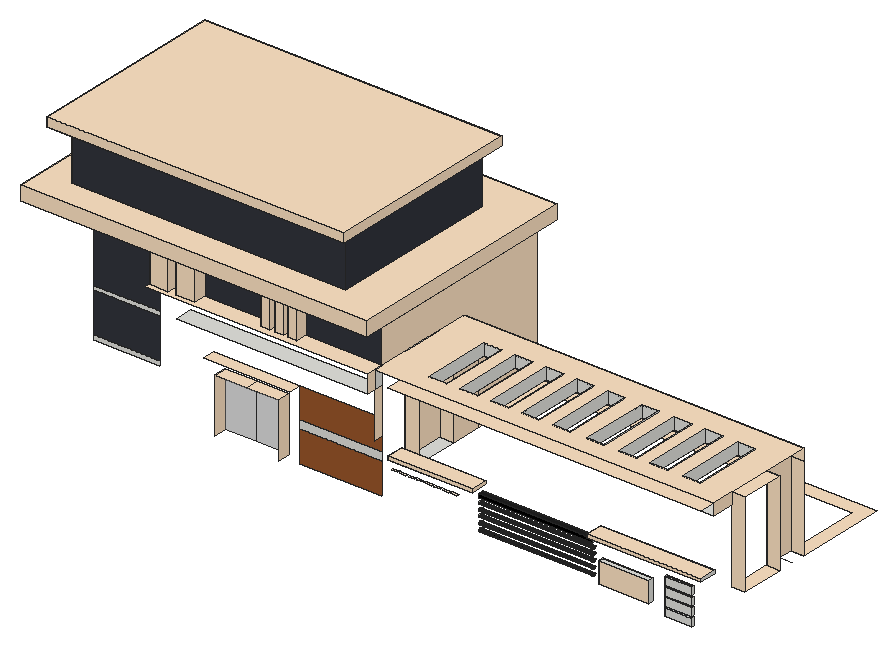
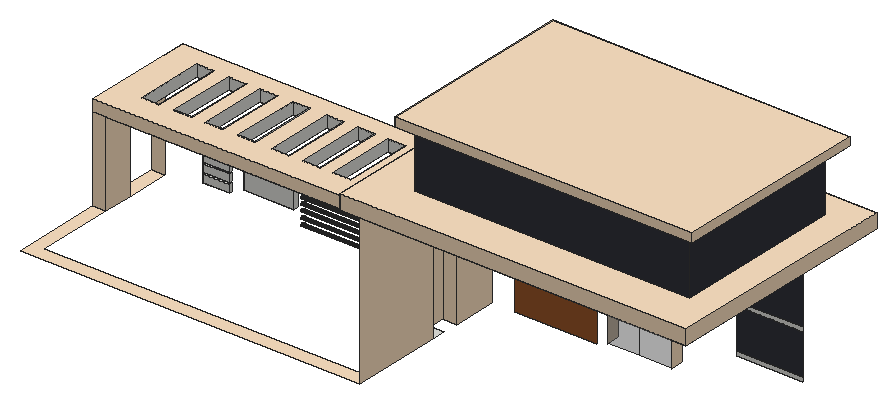
# SketchUp Ruby script. Lengths in inches.
U = 1.inch
M = Sketchup.active_model
def pt(a) = Geom::Point3d.new(a.map { |v| v * U })
def face(e, loops, mat)
  f = e.add_face(loops[0].map { |a| pt(a) })
  loops[1..].each { |l| e.add_face(l.map { |a| pt(a) }).erase! }
  f.material = f.back_material = mat if mat
  f
end
# faces: each face lists its corners as indices into pts; further lists are holes
def faces(e, pts, list, mat = nil) = list.each { |f| face(e, (f[0].is_a?(Array) ? f : [f]).map { |l| l.map { |i| pts[i] } }, mat) }
# xy, xz, yz: faces in a plane at the given z, y or x. An outline is a flat list of corners, or four numbers for a rectangle; further outlines are holes
def ring(l) = l.size == 4 ? [[l[0], l[1]], [l[2], l[1]], [l[2], l[3]], [l[0], l[3]]] : l.each_slice(2).to_a
def flat(e, list, mat, &to3) = list.each { |f| face(e, (f[0].is_a?(Array) ? f : [f]).map { |l| ring(l).map { |u, v| to3.(u, v) } }, mat) }
def xy(e, z, list, mat = nil) = flat(e, list, mat) { |x, y| [x, y, z] }
def xz(e, y, list, mat = nil) = flat(e, list, mat) { |x, z| [x, y, z] }
def yz(e, x, list, mat = nil) = flat(e, list, mat) { |y, z| [x, y, z] }
def lines(e, pts, list) = list.each { |a, b| e.add_line(pt(pts[a]), pt(pts[b])) }
# prism: a flat outline (further loops are holes) pulled along v
def prism(e, loops, v, mat = nil)
  f = face(e, loops, mat); d = Geom::Vector3d.new(v.map { |x| x * U })
  f.pushpull(f.normal.samedirection?(d) ? d.length : -d.length)
end
def box(e, o, s, mat = nil) = prism(e, [[o, [o[0] + s[0], o[1], o[2]], [o[0] + s[0], o[1] + s[1], o[2]], [o[0], o[1] + s[1], o[2]]]], [0, 0, s[2]], mat)
def at(x, y, z, deg = 0) = Geom::Transformation.translation(pt([x, y, z])) * Geom::Transformation.rotation(ORIGIN, Z_AXIS, deg.degrees)
def axes(o, x, y, z) = Geom::Transformation.new([*x, 0, *y, 0, *z, 0, *pt(o).to_a, 1])
def part(name) = M.definitions.add(name)
# library, detail: a bought-in or finely detailed component or shape, given as its bounding box
def library(name, o, s) = part(name).tap { |d| box(d.entities, o, s) }
def detail(e, o, s) = box(e.add_group.entities, o, s)
def put(e, d, t, mat = nil) = e.add_instance(d, t).tap { |i| i.material = mat if mat }
def group(e, t, mat = nil) = e.add_group.tap { |g| g.transformation = t; g.material = mat if mat }.entities
root = M.entities
M.materials.add("[0012_Bisque]").color = [255, 228, 196]
M.materials.add("[0028_AntiqueWhite]").color = [250, 235, 215]
M.materials.add("[Color M08]").color = [30, 30, 30]
M.materials.add("[Color M09]").color = [0, 0, 0]
M.materials.add("[Formica Laminate Dark]").color = [50, 53, 60]
M.materials.add("[Translucent Glass Gray]").color = [128, 128, 128]
M.materials["[Translucent Glass Gray]"].alpha = 0.5
M.materials.add("[Wood Cherry Original]").color = [152, 86, 42]
box(root,[407.7,39.05,294.93],[17.88,1.62,5])
box(root,[407.7,39.05,301.12],[17.88,1.62,5])
box(root,[407.7,39.05,307.12],[17.88,1.62,5])
box(root,[407.7,39.05,313.43],[17.88,1.62,5])
xy(root,300,[[365.58,37.23,398.96,40.67]])
xy(root,308.625,[[215,65.9,223.75,94.79],[215,105.21,223.75,114.71]])
xy(root,308.625,[[430.46,65.9,439.21,94.79],[215,114.71,223.75,114.71,223.75,165.7,430.46,165.7,430.46,114.71,439.21,114.71,439.21,174.44,215,174.44]],"[0012_Bisque]")
xy(root,313.68,[[365.58,37.23,398.96,40.67]])
xy(root,317.125,[[[279.65,45.65,355.06,49.39],[330.07,45.65,330.29,45.68,330.5,45.77,330.68,45.91,330.82,46.09,330.91,46.3,330.94,46.53,330.91,46.75,330.82,46.96,330.68,47.15,330.5,47.29,330.29,47.37,330.07,47.4,329.84,47.37,329.63,47.29,329.45,47.15,329.31,46.96,329.22,46.75,329.19,46.53,329.22,46.3,329.31,46.09,329.45,45.91,329.63,45.77,329.84,45.68],[305.63,45.65,305.85,45.68,306.07,45.77,306.25,45.91,306.39,46.09,306.47,46.3,306.5,46.53,306.47,46.75,306.39,46.96,306.25,47.15,306.07,47.29,305.85,47.37,305.63,47.4,305.4,47.37,305.19,47.29,305.01,47.15,304.87,46.96,304.78,46.75,304.75,46.53,304.78,46.3,304.87,46.09,305.01,45.91,305.19,45.77,305.4,45.68]]],"[Color M08]")
xy(root,317.98,[[227.14,39.36,231.39,40.67],[232.64,39.36,236.89,40.67],[238.51,39.36,242.76,40.67],[244.08,39.36,248.33,40.67],[249.76,39.36,254.01,40.67],
  [255.33,39.36,259.58,40.67],[260.95,39.36,265.2,40.67],[266.39,39.36,270.64,40.67]],"[0028_AntiqueWhite]")
xy(root,319.4375,[[279.65,45.65,355.06,49.39]],"[Color M08]")
xy(root,322.3125,[[223.75,40.67,279.65,51.97],[355.06,40.67,430.46,51.97]])
xy(root,324.5,[[223.75,40.67,279.65,51.97],[355.06,40.67,430.46,51.97]],"[0012_Bisque]")
xy(root,333.89,[[111.55,38.36,132.61,46.73],[132.61,38.36,153.67,46.73]],"[0012_Bisque]")
xy(root,341.36,[[104.08,38.36,161.14,46.73]],"[0012_Bisque]")
xy(root,360.6,[[89.06,35.36,215,46.73]])
xy(root,364.53,[[430.46,40.67,439.21,55.48]])
xy(root,364.53,[[[223.75,40.67,223.75,65.9,215,65.9,215,94.79,223.75,94.79,223.75,114.71,430.46,114.71,430.46,94.79,439.21,94.79,439.21,65.9,430.46,65.9,430.46,40.67],[241.35,52.73,252.92,98.23],[408.67,52.73,420.23,98.23],[261.85,52.73,273.42,98.23],[387.17,52.73,398.73,98.23],[282.29,52.73,293.85,98.23],[366.79,52.73,378.35,98.23],[302.29,52.73,313.85,98.23],[345.29,52.73,356.85,98.23],[322.73,52.73,334.29,98.23]]],"[0012_Bisque]")
xy(root,372.25,[[68.38,38.48,80.44,46.73],[85.88,38.48,97.94,46.73],[140.45,39.92,146.58,46.73],[149.51,39.92,155.64,46.73],[158.39,39.92,164.51,46.73]])
xy(root,372.25,[[68.38,35.36,215,35.36,215,46.73,164.51,46.73,164.51,39.92,158.39,39.92,158.39,46.73,155.64,46.73,155.64,39.92,149.51,39.92,149.51,46.73,146.58,46.73,146.58,39.92,140.45,39.92,140.45,46.73,97.94,46.73,97.94,38.48,85.88,38.48,85.88,46.73,80.44,46.73,80.44,38.48,68.38,38.48],[[215,40.67,439.21,114.71],[241.35,52.73,252.92,98.23],[261.85,52.73,273.42,98.23],[282.29,52.73,293.85,98.23],[302.29,52.73,313.85,98.23],[322.73,52.73,334.29,98.23],[345.29,52.73,356.85,98.23],[366.79,52.73,378.35,98.23],[387.17,52.73,398.73,98.23],[408.67,52.73,420.23,98.23]]],"[0012_Bisque]")
xy(root,397.4375,[[68.38,38.48,80.44,46.73],[85.88,38.48,97.94,46.73]],"[0012_Bisque]")
xy(root,398.3125,[[140.45,39.92,146.58,46.73],[149.51,39.92,155.64,46.73],[158.39,39.92,164.51,46.73]],"[0012_Bisque]")
xy(root,406.75,[[24.6875,46.73,215,174.44]])
xy(root,406.75,[[0,17.17,228.57,46.73],[0,46.73,24.6875,174.44],[215,46.73,228.57,174.44]],"[0012_Bisque]")
xy(root,416.3125,[[18.79,35.8,200.11,147.86]])
xy(root,416.3125,[[[0,17.17,228.57,174.44],[18.79,35.8,200.11,147.86]]],"[0012_Bisque]")
xy(root,453.1875,[[13.16,22.61,209.05,35.8],[13.16,35.8,18.79,147.86],[18.79,35.8,200.11,147.86],[200.11,35.8,209.05,152.92],[13.16,147.86,200.11,152.92]])
xy(root,459,[[13.16,22.61,209.05,152.92]],"[0012_Bisque]")
xz(root,17.17,[[0,406.75,228.57,416.3125]],"[0012_Bisque]")
xz(root,22.61,[[13.16,453.1875,209.05,459]],"[0012_Bisque]")
xz(root,35.8,[[18.79,416.3125,200.11,453.1875]],"[Formica Laminate Dark]")
xz(root,37.23,[[365.58,300,398.96,313.68]],"[0012_Bisque]")
xz(root,38.48,[[68.38,372.25,80.44,397.4375],[85.88,372.25,97.94,397.4375]],"[0012_Bisque]")
xz(root,39.92,[[140.45,372.25,146.58,398.3125],[149.51,372.25,155.64,398.3125],[158.39,372.25,164.51,398.3125]],"[0012_Bisque]")
xz(root,40.67,[[365.58,300,398.96,313.68]])
xz(root,40.67,[[223.75,322.3125,279.65,324.5],[355.06,322.3125,430.46,324.5]],"[0012_Bisque]")
xz(root,45.65,[[279.65,317.125,355.06,319.4375]],"[Color M09]")
xz(root,46.73,[[161.14,315.73,215,320.89],[24.6875,320.49,68.38,323.52],[24.6875,349.9375,68.38,352.67],[68.38,372.25,80.44,397.4375],[85.88,372.25,97.94,397.4375],
  [140.45,372.25,146.58,398.3125],[149.51,372.25,155.64,398.3125],[158.39,372.25,164.51,398.3125]])
xz(root,46.73,[[24.6875,323.52,68.38,349.9375],[24.6875,352.67,68.38,352.67,68.38,397.4375,80.44,397.4375,80.44,372.25,85.88,372.25,85.88,397.4375,97.94,397.4375,97.94,372.25,140.45,372.25,140.45,398.3125,146.58,398.3125,146.58,372.25,149.51,372.25,149.51,398.3125,155.64,398.3125,155.64,372.25,158.39,372.25,158.39,398.3125,164.51,398.3125,164.51,372.25,215,372.25,215,406.75,24.6875,406.75]],"[Formica Laminate Dark]")
xz(root,46.73,[[111.55,297.86,132.61,333.89],[132.61,297.86,153.67,333.89]],"[Translucent Glass Gray]")
xz(root,46.73,[[161.14,295.26,215,315.73],[161.14,320.89,215,341.36]],"[Wood Cherry Original]")
xz(root,49.39,[[279.65,317.125,355.06,319.4375]],"[Formica Laminate Dark]")
xz(root,51.97,[[223.75,322.3125,279.65,324.5],[355.06,322.3125,430.46,324.5]],"[0012_Bisque]")
xz(root,52.73,[[241.35,364.53,252.92,372.25],[261.85,364.53,273.42,372.25],[282.29,364.53,293.85,372.25],[302.29,364.53,313.85,372.25],[322.73,364.53,334.29,372.25],
  [345.29,364.53,356.85,372.25],[366.79,364.53,378.35,372.25],[387.17,364.53,398.73,372.25],[408.67,364.53,420.23,372.25]])
xz(root,65.9,[[215,308.625,223.75,364.53],[430.46,308.625,439.21,364.53]],"[0012_Bisque]")
xz(root,94.79,[[215,308.625,223.75,364.53],[430.46,308.625,439.21,364.53]],"[0012_Bisque]")
xz(root,98.23,[[241.35,364.53,252.92,372.25],[261.85,364.53,273.42,372.25],[282.29,364.53,293.85,372.25],[302.29,364.53,313.85,372.25],[322.73,364.53,334.29,372.25],
  [345.29,364.53,356.85,372.25],[366.79,364.53,378.35,372.25],[387.17,364.53,398.73,372.25],[408.67,364.53,420.23,372.25]])
xz(root,114.71,[[215,308.625,215,372.25,439.21,372.25,439.21,364.53,223.75,364.53,223.75,308.625],[430.46,308.625,439.21,364.53]],"[0012_Bisque]")
xz(root,147.86,[[18.79,416.3125,200.11,453.1875]],"[Formica Laminate Dark]")
xz(root,152.92,[[13.16,453.1875,209.05,459]],"[0012_Bisque]")
xz(root,174.44,[[0,406.75,228.57,416.3125]],"[0012_Bisque]")
yz(root,0,[[17.17,406.75,174.44,416.3125]],"[0012_Bisque]")
yz(root,13.16,[[22.61,453.1875,152.92,459]],"[0012_Bisque]")
yz(root,18.79,[[35.8,416.3125,147.86,453.1875]],"[Formica Laminate Dark]")
yz(root,68.38,[[38.48,372.25,46.73,397.4375]],"[0012_Bisque]")
yz(root,80.44,[[38.48,372.25,46.73,397.4375]],"[0012_Bisque]")
yz(root,85.88,[[38.48,372.25,46.73,397.4375]],"[0012_Bisque]")
yz(root,97.94,[[38.48,372.25,46.73,397.4375]],"[0012_Bisque]")
yz(root,111.55,[[38.36,297.86,46.73,333.89]],"[0012_Bisque]")
yz(root,140.45,[[39.92,372.25,46.73,398.3125]],"[0012_Bisque]")
yz(root,146.58,[[39.92,372.25,46.73,398.3125]],"[0012_Bisque]")
yz(root,149.51,[[39.92,372.25,46.73,398.3125]],"[0012_Bisque]")
yz(root,153.67,[[38.36,297.86,46.73,333.89]],"[0012_Bisque]")
yz(root,155.64,[[39.92,372.25,46.73,398.3125]],"[0012_Bisque]")
yz(root,158.39,[[39.92,372.25,46.73,398.3125]],"[0012_Bisque]")
yz(root,164.51,[[39.92,372.25,46.73,398.3125]],"[0012_Bisque]")
yz(root,200.11,[[35.8,416.3125,147.86,453.1875]],"[Formica Laminate Dark]")
yz(root,209.05,[[22.61,453.1875,152.92,459]],"[0012_Bisque]")
yz(root,215,[[40.67,360.6,46.73,372.25],[65.9,364.53,94.79,372.25]])
yz(root,215,[[114.71,308.625,174.44,308.625,174.44,406.75,46.73,406.75,46.73,372.25,114.71,372.25],[65.9,308.625,94.79,364.53],[40.67,330.3125,46.73,360.6],[35.36,360.6,40.67,372.25]],"[0012_Bisque]")
yz(root,223.75,[[40.67,322.3125,51.97,324.5]])
yz(root,223.75,[[94.79,308.625,114.71,364.53]],"[0012_Bisque]")
yz(root,228.57,[[17.17,406.75,174.44,416.3125]],"[0012_Bisque]")
yz(root,241.35,[[52.73,364.53,98.23,372.25]])
yz(root,252.92,[[52.73,364.53,98.23,372.25]])
yz(root,261.85,[[52.73,364.53,98.23,372.25]])
yz(root,273.42,[[52.73,364.53,98.23,372.25]])
yz(root,279.65,[[46.99,296.71,46.77,296.74,46.55,296.83,46.375,296.97,46.23,297.15,46.15,297.36,46.12,297.59,46.15,297.8125,46.23,298.02,46.375,298.2,46.55,298.34,46.77,298.43,46.99,298.46,47.22,298.43,47.43,298.34,47.61,298.2,47.75,298.02,47.84,297.8125,47.87,297.59,47.84,297.36,47.75,297.15,47.61,296.97,47.43,296.83,47.22,296.74],[46.99,300.84,46.77,300.87,46.55,300.95,46.375,301.09,46.23,301.27,46.15,301.48,46.12,301.71,46.15,301.9375,46.23,302.15,46.375,302.33,46.55,302.47,46.77,302.56,46.99,302.59,47.22,302.56,47.43,302.47,47.61,302.33,47.75,302.15,47.84,301.9375,47.87,301.71,47.84,301.48,47.75,301.27,47.61,301.09,47.43,300.95,47.22,300.87],[46.99,305.27,46.77,305.3,46.55,305.39,46.375,305.53,46.23,305.71,46.15,305.92,46.12,306.15,46.15,306.375,46.23,306.59,46.375,306.77,46.55,306.91,46.77,306.99,46.99,307.02,47.22,306.99,47.43,306.91,47.61,306.77,47.75,306.59,47.84,306.375,47.87,306.15,47.84,305.92,47.75,305.71,47.61,305.53,47.43,305.39,47.22,305.3],[46.99,308.96,46.77,308.99,46.55,309.08,46.375,309.22,46.23,309.4,46.15,309.61,46.12,309.84,46.15,310.0625,46.23,310.27,46.375,310.45,46.55,310.59,46.77,310.68,46.99,310.71,47.22,310.68,47.43,310.59,47.61,310.45,47.75,310.27,47.84,310.0625,47.87,309.84,47.84,309.61,47.75,309.4,47.61,309.22,47.43,309.08,47.22,308.99],[46.99,313.02,46.77,313.05,46.55,313.14,46.375,313.28,46.23,313.46,46.15,313.67,46.12,313.9,46.15,314.125,46.23,314.34,46.375,314.52,46.55,314.66,46.77,314.74,46.99,314.77,47.22,314.74,47.43,314.66,47.61,314.52,47.75,314.34,47.84,314.125,47.87,313.9,47.84,313.67,47.75,313.46,47.61,313.28,47.43,313.14,47.22,313.05]])
yz(root,279.65,[[40.67,322.3125,51.97,324.5]],"[0012_Bisque]")
yz(root,282.29,[[52.73,364.53,98.23,372.25]])
yz(root,293.85,[[52.73,364.53,98.23,372.25]])
yz(root,302.29,[[52.73,364.53,98.23,372.25]])
yz(root,313.85,[[52.73,364.53,98.23,372.25]])
yz(root,322.73,[[52.73,364.53,98.23,372.25]])
yz(root,334.29,[[52.73,364.53,98.23,372.25]])
yz(root,345.29,[[52.73,364.53,98.23,372.25]])
yz(root,355.06,[[45.65,317.125,49.39,319.4375]])
yz(root,355.06,[[40.67,322.3125,51.97,324.5]],"[0012_Bisque]")
yz(root,356.85,[[52.73,364.53,98.23,372.25]])
yz(root,365.58,[[37.23,300,40.67,313.68]])
yz(root,366.79,[[52.73,364.53,98.23,372.25]])
yz(root,378.35,[[52.73,364.53,98.23,372.25]])
yz(root,387.17,[[52.73,364.53,98.23,372.25]])
yz(root,398.73,[[52.73,364.53,98.23,372.25]])
yz(root,398.96,[[37.23,300,40.67,313.68]])
yz(root,408.67,[[52.73,364.53,98.23,372.25]])
yz(root,420.23,[[52.73,364.53,98.23,372.25]])
yz(root,430.46,[[40.67,322.3125,51.97,324.5]])
yz(root,430.46,[[94.79,308.625,114.71,364.53]],"[0012_Bisque]")
yz(root,439.21,[[40.67,364.53,55.48,372.25]],"[0012_Bisque]")
p = [[279.65,46.55,296.83],[279.65,46.77,296.74],[355.06,46.77,296.74],[355.06,46.55,296.83],[279.65,46.99,296.71],[355.06,46.99,296.71],
  [279.65,47.22,296.74],[355.06,47.22,296.74],[279.65,47.43,296.83],[355.06,47.43,296.83],[279.65,46.375,296.97],[355.06,46.375,296.97],
  [279.65,47.61,296.97],[355.06,47.61,296.97],[279.65,46.23,297.15],[355.06,46.23,297.15],[279.65,47.75,297.15],[355.06,47.75,297.15],
  [279.65,46.15,297.36],[355.06,46.15,297.36],[279.65,47.84,297.36],[355.06,47.84,297.36],[279.65,46.12,297.59],[355.06,46.12,297.59],
  [279.65,47.87,297.59],[355.06,47.87,297.59],[279.65,46.15,297.8125],[355.06,46.15,297.8125],[279.65,47.84,297.8125],[355.06,47.84,297.8125],
  [279.65,46.23,298.02],[355.06,46.23,298.02],[279.65,47.75,298.02],[355.06,47.75,298.02],[279.65,46.375,298.2],[355.06,46.375,298.2],
  [279.65,47.61,298.2],[355.06,47.61,298.2],[279.65,46.55,298.34],[355.06,46.55,298.34],[279.65,47.43,298.34],[355.06,47.43,298.34],
  [279.65,46.77,298.43],[355.06,46.77,298.43],[279.65,47.22,298.43],[355.06,47.22,298.43],[279.65,46.99,298.46],[355.06,46.99,298.46],
  [279.65,46.77,300.87],[279.65,46.99,300.84],[355.06,46.99,300.84],[355.06,46.77,300.87],[279.65,47.22,300.87],[355.06,47.22,300.87],
  [279.65,46.55,300.95],[355.06,46.55,300.95],[279.65,47.43,300.95],[355.06,47.43,300.95],[279.65,46.375,301.09],[355.06,46.375,301.09],
  [279.65,47.61,301.09],[355.06,47.61,301.09],[279.65,46.23,301.27],[355.06,46.23,301.27],[279.65,47.75,301.27],[355.06,47.75,301.27],
  [279.65,46.15,301.48],[355.06,46.15,301.48],[279.65,47.84,301.48],[355.06,47.84,301.48],[279.65,46.12,301.71],[355.06,46.12,301.71],
  [279.65,47.87,301.71],[355.06,47.87,301.71],[279.65,46.15,301.9375],[355.06,46.15,301.9375],[279.65,47.84,301.9375],[355.06,47.84,301.9375],
  [279.65,46.23,302.15],[355.06,46.23,302.15],[279.65,47.75,302.15],[355.06,47.75,302.15],[279.65,46.375,302.33],[355.06,46.375,302.33],
  [279.65,47.61,302.33],[355.06,47.61,302.33],[279.65,46.55,302.47],[355.06,46.55,302.47],[279.65,47.43,302.47],[355.06,47.43,302.47],
  [279.65,46.77,302.56],[355.06,46.77,302.56],[279.65,47.22,302.56],[355.06,47.22,302.56],[279.65,46.99,302.59],[355.06,46.99,302.59],
  [279.65,46.55,305.39],[279.65,46.77,305.3],[355.06,46.77,305.3],[355.06,46.55,305.39],[279.65,46.99,305.27],[355.06,46.99,305.27],
  [279.65,47.22,305.3],[355.06,47.22,305.3],[279.65,47.43,305.39],[355.06,47.43,305.39],[279.65,46.375,305.53],[355.06,46.375,305.53],
  [279.65,47.61,305.53],[355.06,47.61,305.53],[279.65,46.23,305.71],[355.06,46.23,305.71],[279.65,47.75,305.71],[355.06,47.75,305.71],
  [279.65,46.15,305.92],[355.06,46.15,305.92],[279.65,47.84,305.92],[355.06,47.84,305.92],[279.65,46.12,306.15],[355.06,46.12,306.15],
  [279.65,47.87,306.15],[355.06,47.87,306.15],[279.65,46.15,306.375],[355.06,46.15,306.375],[279.65,47.84,306.375],[355.06,47.84,306.375],
  [279.65,46.23,306.59],[355.06,46.23,306.59],[279.65,47.75,306.59],[355.06,47.75,306.59],[279.65,46.375,306.77],[355.06,46.375,306.77],
  [279.65,47.61,306.77],[355.06,47.61,306.77],[279.65,46.55,306.91],[355.06,46.55,306.91],[279.65,47.43,306.91],[355.06,47.43,306.91],
  [279.65,46.77,306.99],[355.06,46.77,306.99],[279.65,47.22,306.99],[355.06,47.22,306.99],[279.65,46.99,307.02],[355.06,46.99,307.02],
  [279.65,46.55,309.08],[279.65,46.77,308.99],[355.06,46.77,308.99],[355.06,46.55,309.08],[279.65,46.99,308.96],[355.06,46.99,308.96],
  [279.65,47.22,308.99],[355.06,47.22,308.99],[279.65,47.43,309.08],[355.06,47.43,309.08],[279.65,46.375,309.22],[355.06,46.375,309.22],
  [279.65,47.61,309.22],[355.06,47.61,309.22],[279.65,46.23,309.4],[355.06,46.23,309.4],[279.65,47.75,309.4],[355.06,47.75,309.4],
  [279.65,46.15,309.61],[355.06,46.15,309.61],[279.65,47.84,309.61],[355.06,47.84,309.61],[279.65,46.12,309.84],[355.06,46.12,309.84],
  [279.65,47.87,309.84],[355.06,47.87,309.84],[279.65,46.15,310.0625],[355.06,46.15,310.0625],[279.65,47.84,310.0625],[355.06,47.84,310.0625],
  [279.65,46.23,310.27],[355.06,46.23,310.27],[279.65,47.75,310.27],[355.06,47.75,310.27],[279.65,46.375,310.45],[355.06,46.375,310.45],
  [279.65,47.61,310.45],[355.06,47.61,310.45],[279.65,46.55,310.59],[355.06,46.55,310.59],[279.65,47.43,310.59],[355.06,47.43,310.59],
  [279.65,46.77,310.68],[355.06,46.77,310.68],[279.65,47.22,310.68],[355.06,47.22,310.68],[279.65,46.99,310.71],[355.06,46.99,310.71],
  [279.65,46.77,313.05],[279.65,46.99,313.02],[355.06,46.99,313.02],[355.06,46.77,313.05],[279.65,47.22,313.05],[355.06,47.22,313.05],
  [279.65,46.375,313.28],[279.65,46.55,313.14],[355.06,46.55,313.14],[355.06,46.375,313.28],[279.65,47.43,313.14],[355.06,47.43,313.14],
  [279.65,47.61,313.28],[355.06,47.61,313.28],[279.65,46.23,313.46],[355.06,46.23,313.46],[279.65,47.75,313.46],[355.06,47.75,313.46],
  [279.65,46.15,313.67],[355.06,46.15,313.67],[279.65,47.84,313.67],[355.06,47.84,313.67],[279.65,46.12,313.9],[355.06,46.12,313.9],
  [279.65,47.87,313.9],[355.06,47.87,313.9],[279.65,46.15,314.125],[355.06,46.15,314.125],[279.65,47.84,314.125],[355.06,47.84,314.125],
  [279.65,46.23,314.34],[355.06,46.23,314.34],[279.65,47.75,314.34],[355.06,47.75,314.34],[279.65,46.375,314.52],[355.06,46.375,314.52],
  [279.65,47.61,314.52],[355.06,47.61,314.52],[279.65,46.55,314.66],[355.06,46.55,314.66],[279.65,47.43,314.66],[355.06,47.43,314.66],
  [279.65,46.77,314.74],[355.06,46.77,314.74],[279.65,46.99,314.77],[355.06,46.99,314.77],[279.65,47.22,314.74],[355.06,47.22,314.74],
  [430.46,105.21,308.625],[439.21,105.21,308.625]]
faces(root,p,[[0,1,2,3],[1,4,5,2],[4,6,7,5],[6,8,9,7],[10,0,3,11],[8,12,13,9],[14,10,11,15],[12,16,17,13],
  [18,14,15,19],[16,20,21,17],[22,18,19,23],[20,24,25,21],[26,22,23,27],[24,28,29,25],[30,26,27,31],[28,32,33,29],
  [34,30,31,35],[32,36,37,33],[38,34,35,39],[36,40,41,37],[42,38,39,43],[40,44,45,41],[46,42,43,47],[44,46,47,45],
  [48,49,50,51],[49,52,53,50],[54,48,51,55],[52,56,57,53],[58,54,55,59],[56,60,61,57],[62,58,59,63],[60,64,65,61],
  [66,62,63,67],[64,68,69,65],[70,66,67,71],[68,72,73,69],[74,70,71,75],[72,76,77,73],[78,74,75,79],[76,80,81,77],
  [82,78,79,83],[80,84,85,81],[86,82,83,87],[84,88,89,85],[90,86,87,91],[88,92,93,89],[94,90,91,95],[92,94,95,93],
  [96,97,98,99],[97,100,101,98],[100,102,103,101],[102,104,105,103],[106,96,99,107],[104,108,109,105],[110,106,107,111],[108,112,113,109],
  [114,110,111,115],[112,116,117,113],[118,114,115,119],[116,120,121,117],[122,118,119,123],[120,124,125,121],[126,122,123,127],[124,128,129,125],
  [130,126,127,131],[128,132,133,129],[134,130,131,135],[132,136,137,133],[138,134,135,139],[136,140,141,137],[142,138,139,143],[140,142,143,141],
  [144,145,146,147],[145,148,149,146],[148,150,151,149],[150,152,153,151],[154,144,147,155],[152,156,157,153],[158,154,155,159],[156,160,161,157],
  [162,158,159,163],[160,164,165,161],[166,162,163,167],[164,168,169,165],[170,166,167,171],[168,172,173,169],[174,170,171,175],[172,176,177,173],
  [178,174,175,179],[176,180,181,177],[182,178,179,183],[180,184,185,181],[186,182,183,187],[184,188,189,185],[190,186,187,191],[188,190,191,189],
  [192,193,194,195],[193,196,197,194],[198,199,200,201],[199,192,195,200],[196,202,203,197],[202,204,205,203],[206,198,201,207],[204,208,209,205],
  [210,206,207,211],[208,212,213,209],[214,210,211,215],[212,216,217,213],[218,214,215,219],[216,220,221,217],[222,218,219,223],[220,224,225,221],
  [226,222,223,227],[224,228,229,225],[230,226,227,231],[228,232,233,229],[234,230,231,235],[236,234,235,237],[238,236,237,239],[232,238,239,233]],"[Color M09]")
lines(root,p,[[240,241]])
